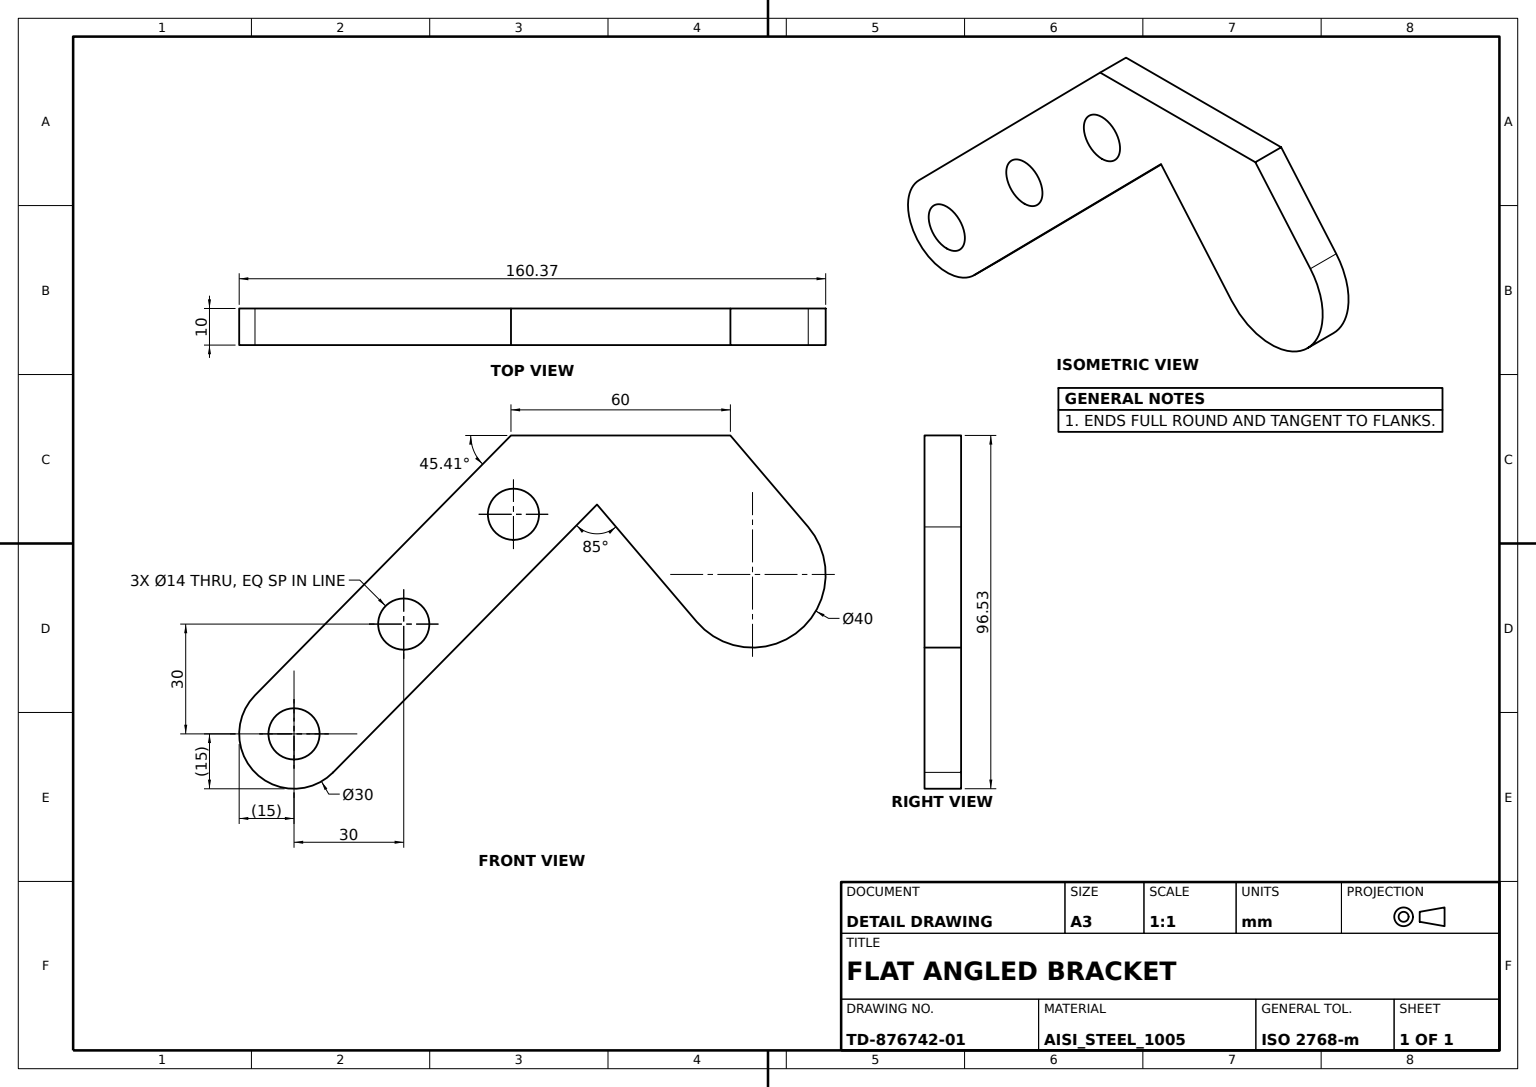
ISO-10303-21;
HEADER;
FILE_DESCRIPTION((''),'2;1');
FILE_NAME('','',(''),(''),'','','');
FILE_SCHEMA(('AUTOMOTIVE_DESIGN'));
ENDSEC;
DATA;
#1=APPLICATION_CONTEXT('');
#2=PRODUCT_CONTEXT('',#1,'mechanical');
#3=PRODUCT('','','',(#2));
#4=PRODUCT_DEFINITION_FORMATION('','',#3);
#5=PRODUCT_DEFINITION_CONTEXT('',#1,'design');
#6=PRODUCT_DEFINITION('','',#4,#5);
#7=PRODUCT_DEFINITION_SHAPE('','',#6);
#8=(LENGTH_UNIT()NAMED_UNIT(*)SI_UNIT(.MILLI.,.METRE.));
#9=(NAMED_UNIT(*)PLANE_ANGLE_UNIT()SI_UNIT($,.RADIAN.));
#10=(NAMED_UNIT(*)SI_UNIT($,.STERADIAN.)SOLID_ANGLE_UNIT());
#11=UNCERTAINTY_MEASURE_WITH_UNIT(LENGTH_MEASURE(0.005),#8,'distance_accuracy_value','');
#12=(GEOMETRIC_REPRESENTATION_CONTEXT(3)GLOBAL_UNCERTAINTY_ASSIGNED_CONTEXT((#11))GLOBAL_UNIT_ASSIGNED_CONTEXT((#8,#9,#10))REPRESENTATION_CONTEXT('',''));
#13=CARTESIAN_POINT('',(-37.964085,-6.052113,10.));
#14=VERTEX_POINT('',#13);
#15=CARTESIAN_POINT('',(-37.964085,-66.052113,10.));
#16=VERTEX_POINT('',#15);
#17=DIRECTION('',(0.,-1.,0.));
#18=VECTOR('',#17,1000.);
#19=LINE('',#13,#18);
#20=EDGE_CURVE('',#14,#16,#19,.T.);
#21=ORIENTED_EDGE('',*,*,#20,.F.);
#22=CARTESIAN_POINT('',(-37.964085,-6.052113,0.));
#23=VERTEX_POINT('',#22);
#24=DIRECTION('',(0.,0.,-1.));
#25=VECTOR('',#24,1000.);
#26=LINE('',#13,#25);
#27=EDGE_CURVE('',#14,#23,#26,.T.);
#28=ORIENTED_EDGE('',*,*,#27,.T.);
#29=CARTESIAN_POINT('',(-37.964085,-66.052113,0.));
#30=VERTEX_POINT('',#29);
#31=LINE('',#22,#18);
#32=EDGE_CURVE('',#23,#30,#31,.T.);
#33=ORIENTED_EDGE('',*,*,#32,.T.);
#34=LINE('',#15,#25);
#35=EDGE_CURVE('',#16,#30,#34,.T.);
#36=ORIENTED_EDGE('',*,*,#35,.F.);
#37=EDGE_LOOP('',(#21,#28,#33,#36));
#38=FACE_BOUND('',#37,.T.);
#39=DIRECTION('',(1.,0.,0.));
#40=AXIS2_PLACEMENT_3D('',#13,#39,#24);
#41=PLANE('',#40);
#42=ADVANCED_FACE('',(#38),#41,.F.);
#43=CARTESIAN_POINT('',(20.567028,-95.370555,0.));
#44=VERTEX_POINT('',#43);
#45=CARTESIAN_POINT('',(13.567028,-95.370555,0.));
#46=DIRECTION('',(0.,0.,1.));
#47=AXIS2_PLACEMENT_3D('',#45,#46,#39);
#48=CIRCLE('',#47,7.);
#49=EDGE_CURVE('',#44,#44,#48,.T.);
#50=ORIENTED_EDGE('',*,*,#49,.T.);
#51=EDGE_LOOP('',(#50));
#52=FACE_BOUND('',#51,.T.);
#53=CARTESIAN_POINT('',(50.567028,-125.370555,0.));
#54=VERTEX_POINT('',#53);
#55=CARTESIAN_POINT('',(43.567028,-125.370555,0.));
#56=AXIS2_PLACEMENT_3D('',#55,#46,#39);
#57=CIRCLE('',#56,7.);
#58=EDGE_CURVE('',#54,#54,#57,.T.);
#59=ORIENTED_EDGE('',*,*,#58,.T.);
#60=EDGE_LOOP('',(#59));
#61=FACE_BOUND('',#60,.T.);
#62=CARTESIAN_POINT('',(-9.432972,-65.370555,0.));
#63=VERTEX_POINT('',#62);
#64=CARTESIAN_POINT('',(-16.432972,-65.370555,0.));
#65=AXIS2_PLACEMENT_3D('',#64,#46,#39);
#66=CIRCLE('',#65,7.);
#67=EDGE_CURVE('',#63,#63,#66,.T.);
#68=ORIENTED_EDGE('',*,*,#67,.T.);
#69=EDGE_LOOP('',(#68));
#70=FACE_BOUND('',#69,.T.);
#71=CARTESIAN_POINT('',(33.035915,-136.052113,0.));
#72=VERTEX_POINT('',#71);
#73=CARTESIAN_POINT('',(54.098141,-114.688998,0.));
#74=VERTEX_POINT('',#73);
#75=CIRCLE('',#56,15.);
#76=EDGE_CURVE('',#72,#74,#75,.T.);
#77=ORIENTED_EDGE('',*,*,#76,.F.);
#78=DIRECTION('',(0.712103814,-0.702074183,0.));
#79=VECTOR('',#78,1000.);
#80=LINE('',#29,#79);
#81=EDGE_CURVE('',#30,#72,#80,.T.);
#82=ORIENTED_EDGE('',*,*,#81,.F.);
#83=ORIENTED_EDGE('',*,*,#32,.F.);
#84=CARTESIAN_POINT('',(-12.964085,15.22933,0.));
#85=VERTEX_POINT('',#84);
#86=DIRECTION('',(-0.761466515,-0.648204247,0.));
#87=VECTOR('',#86,1000.);
#88=LINE('',#84,#87);
#89=EDGE_CURVE('',#85,#23,#88,.T.);
#90=ORIENTED_EDGE('',*,*,#89,.F.);
#91=CARTESIAN_POINT('',(12.964085,-15.22933,0.));
#92=VERTEX_POINT('',#91);
#93=CARTESIAN_POINT('',(0.,0.,0.));
#94=AXIS2_PLACEMENT_3D('',#93,#46,#39);
#95=CIRCLE('',#94,20.);
#96=EDGE_CURVE('',#92,#85,#95,.T.);
#97=ORIENTED_EDGE('',*,*,#96,.F.);
#98=CARTESIAN_POINT('',(-19.098741,-42.523058,0.));
#99=VERTEX_POINT('',#98);
#100=DIRECTION('',(0.761466515,0.648204247,0.));
#101=VECTOR('',#100,1000.);
#102=LINE('',#98,#101);
#103=EDGE_CURVE('',#99,#92,#102,.T.);
#104=ORIENTED_EDGE('',*,*,#103,.F.);
#105=DIRECTION('',(-0.712103814,0.702074183,0.));
#106=VECTOR('',#105,1000.);
#107=LINE('',#73,#106);
#108=EDGE_CURVE('',#74,#99,#107,.T.);
#109=ORIENTED_EDGE('',*,*,#108,.F.);
#110=EDGE_LOOP('',(#77,#82,#83,#90,#97,#104,#109));
#111=FACE_BOUND('',#110,.T.);
#112=PLANE('',#94);
#113=ADVANCED_FACE('',(#52,#61,#70,#111),#112,.F.);
#114=CARTESIAN_POINT('',(54.098141,-114.688998,10.));
#115=VERTEX_POINT('',#114);
#116=CARTESIAN_POINT('',(-19.098741,-42.523058,10.));
#117=VERTEX_POINT('',#116);
#118=LINE('',#114,#106);
#119=EDGE_CURVE('',#115,#117,#118,.T.);
#120=ORIENTED_EDGE('',*,*,#119,.T.);
#121=CARTESIAN_POINT('',(12.964085,-15.22933,10.));
#122=VERTEX_POINT('',#121);
#123=LINE('',#116,#101);
#124=EDGE_CURVE('',#117,#122,#123,.T.);
#125=ORIENTED_EDGE('',*,*,#124,.T.);
#126=CARTESIAN_POINT('',(-12.964085,15.22933,10.));
#127=VERTEX_POINT('',#126);
#128=CARTESIAN_POINT('',(0.,0.,10.));
#129=AXIS2_PLACEMENT_3D('',#128,#46,#39);
#130=CIRCLE('',#129,20.);
#131=EDGE_CURVE('',#122,#127,#130,.T.);
#132=ORIENTED_EDGE('',*,*,#131,.T.);
#133=LINE('',#126,#87);
#134=EDGE_CURVE('',#127,#14,#133,.T.);
#135=ORIENTED_EDGE('',*,*,#134,.T.);
#136=ORIENTED_EDGE('',*,*,#20,.T.);
#137=CARTESIAN_POINT('',(33.035915,-136.052113,10.));
#138=VERTEX_POINT('',#137);
#139=LINE('',#15,#79);
#140=EDGE_CURVE('',#16,#138,#139,.T.);
#141=ORIENTED_EDGE('',*,*,#140,.T.);
#142=CARTESIAN_POINT('',(43.567028,-125.370555,10.));
#143=AXIS2_PLACEMENT_3D('',#142,#46,#39);
#144=CIRCLE('',#143,15.);
#145=EDGE_CURVE('',#138,#115,#144,.T.);
#146=ORIENTED_EDGE('',*,*,#145,.T.);
#147=EDGE_LOOP('',(#120,#125,#132,#135,#136,#141,#146));
#148=FACE_BOUND('',#147,.T.);
#149=CARTESIAN_POINT('',(-9.432972,-65.370555,10.));
#150=VERTEX_POINT('',#149);
#151=CARTESIAN_POINT('',(-16.432972,-65.370555,10.));
#152=AXIS2_PLACEMENT_3D('',#151,#46,#39);
#153=CIRCLE('',#152,7.);
#154=EDGE_CURVE('',#150,#150,#153,.T.);
#155=ORIENTED_EDGE('',*,*,#154,.F.);
#156=EDGE_LOOP('',(#155));
#157=FACE_BOUND('',#156,.T.);
#158=CARTESIAN_POINT('',(50.567028,-125.370555,10.));
#159=VERTEX_POINT('',#158);
#160=CIRCLE('',#143,7.);
#161=EDGE_CURVE('',#159,#159,#160,.T.);
#162=ORIENTED_EDGE('',*,*,#161,.F.);
#163=EDGE_LOOP('',(#162));
#164=FACE_BOUND('',#163,.T.);
#165=CARTESIAN_POINT('',(20.567028,-95.370555,10.));
#166=VERTEX_POINT('',#165);
#167=CARTESIAN_POINT('',(13.567028,-95.370555,10.));
#168=AXIS2_PLACEMENT_3D('',#167,#46,#39);
#169=CIRCLE('',#168,7.);
#170=EDGE_CURVE('',#166,#166,#169,.T.);
#171=ORIENTED_EDGE('',*,*,#170,.F.);
#172=EDGE_LOOP('',(#171));
#173=FACE_BOUND('',#172,.T.);
#174=PLANE('',#129);
#175=ADVANCED_FACE('',(#148,#157,#164,#173),#174,.T.);
#176=ORIENTED_EDGE('',*,*,#161,.T.);
#177=EDGE_LOOP('',(#176));
#178=FACE_BOUND('',#177,.T.);
#179=ORIENTED_EDGE('',*,*,#58,.F.);
#180=EDGE_LOOP('',(#179));
#181=FACE_BOUND('',#180,.T.);
#182=DIRECTION('',(-1.,0.,0.));
#183=AXIS2_PLACEMENT_3D('',#142,#24,#182);
#184=CYLINDRICAL_SURFACE('',#183,7.);
#185=ADVANCED_FACE('',(#178,#181),#184,.F.);
#186=ORIENTED_EDGE('',*,*,#49,.F.);
#187=EDGE_LOOP('',(#186));
#188=FACE_BOUND('',#187,.T.);
#189=ORIENTED_EDGE('',*,*,#170,.T.);
#190=EDGE_LOOP('',(#189));
#191=FACE_BOUND('',#190,.T.);
#192=AXIS2_PLACEMENT_3D('',#167,#24,#182);
#193=CYLINDRICAL_SURFACE('',#192,7.);
#194=ADVANCED_FACE('',(#188,#191),#193,.F.);
#195=LINE('',#121,#25);
#196=EDGE_CURVE('',#122,#92,#195,.T.);
#197=ORIENTED_EDGE('',*,*,#196,.T.);
#198=ORIENTED_EDGE('',*,*,#96,.T.);
#199=LINE('',#126,#25);
#200=EDGE_CURVE('',#127,#85,#199,.T.);
#201=ORIENTED_EDGE('',*,*,#200,.F.);
#202=ORIENTED_EDGE('',*,*,#131,.F.);
#203=EDGE_LOOP('',(#197,#198,#201,#202));
#204=FACE_BOUND('',#203,.T.);
#205=AXIS2_PLACEMENT_3D('',#128,#24,#182);
#206=CYLINDRICAL_SURFACE('',#205,20.);
#207=ADVANCED_FACE('',(#204),#206,.T.);
#208=LINE('',#114,#25);
#209=EDGE_CURVE('',#115,#74,#208,.T.);
#210=ORIENTED_EDGE('',*,*,#209,.T.);
#211=ORIENTED_EDGE('',*,*,#108,.T.);
#212=LINE('',#116,#25);
#213=EDGE_CURVE('',#117,#99,#212,.T.);
#214=ORIENTED_EDGE('',*,*,#213,.F.);
#215=ORIENTED_EDGE('',*,*,#119,.F.);
#216=EDGE_LOOP('',(#210,#211,#214,#215));
#217=FACE_BOUND('',#216,.T.);
#218=DIRECTION('',(-0.702074183,-0.712103814,0.));
#219=AXIS2_PLACEMENT_3D('',#114,#218,#78);
#220=PLANE('',#219);
#221=ADVANCED_FACE('',(#217),#220,.F.);
#222=ORIENTED_EDGE('',*,*,#124,.F.);
#223=ORIENTED_EDGE('',*,*,#213,.T.);
#224=ORIENTED_EDGE('',*,*,#103,.T.);
#225=ORIENTED_EDGE('',*,*,#196,.F.);
#226=EDGE_LOOP('',(#222,#223,#224,#225));
#227=FACE_BOUND('',#226,.T.);
#228=DIRECTION('',(-0.648204247,0.761466515,0.));
#229=AXIS2_PLACEMENT_3D('',#116,#228,#86);
#230=PLANE('',#229);
#231=ADVANCED_FACE('',(#227),#230,.F.);
#232=ORIENTED_EDGE('',*,*,#89,.T.);
#233=ORIENTED_EDGE('',*,*,#27,.F.);
#234=ORIENTED_EDGE('',*,*,#134,.F.);
#235=ORIENTED_EDGE('',*,*,#200,.T.);
#236=EDGE_LOOP('',(#232,#233,#234,#235));
#237=FACE_BOUND('',#236,.T.);
#238=DIRECTION('',(0.648204247,-0.761466515,0.));
#239=AXIS2_PLACEMENT_3D('',#126,#238,#100);
#240=PLANE('',#239);
#241=ADVANCED_FACE('',(#237),#240,.F.);
#242=ORIENTED_EDGE('',*,*,#67,.F.);
#243=EDGE_LOOP('',(#242));
#244=FACE_BOUND('',#243,.T.);
#245=ORIENTED_EDGE('',*,*,#154,.T.);
#246=EDGE_LOOP('',(#245));
#247=FACE_BOUND('',#246,.T.);
#248=AXIS2_PLACEMENT_3D('',#151,#24,#182);
#249=CYLINDRICAL_SURFACE('',#248,7.);
#250=ADVANCED_FACE('',(#244,#247),#249,.F.);
#251=LINE('',#137,#25);
#252=EDGE_CURVE('',#138,#72,#251,.T.);
#253=ORIENTED_EDGE('',*,*,#252,.T.);
#254=ORIENTED_EDGE('',*,*,#76,.T.);
#255=ORIENTED_EDGE('',*,*,#209,.F.);
#256=ORIENTED_EDGE('',*,*,#145,.F.);
#257=EDGE_LOOP('',(#253,#254,#255,#256));
#258=FACE_BOUND('',#257,.T.);
#259=CYLINDRICAL_SURFACE('',#183,15.);
#260=ADVANCED_FACE('',(#258),#259,.T.);
#261=ORIENTED_EDGE('',*,*,#81,.T.);
#262=ORIENTED_EDGE('',*,*,#252,.F.);
#263=ORIENTED_EDGE('',*,*,#140,.F.);
#264=ORIENTED_EDGE('',*,*,#35,.T.);
#265=EDGE_LOOP('',(#261,#262,#263,#264));
#266=FACE_BOUND('',#265,.T.);
#267=DIRECTION('',(0.702074183,0.712103814,0.));
#268=AXIS2_PLACEMENT_3D('',#15,#267,#105);
#269=PLANE('',#268);
#270=ADVANCED_FACE('',(#266),#269,.F.);
#271=CLOSED_SHELL('',(#42,#113,#175,#185,#194,#207,#221,#231,#241,#250,#260,#270));
#272=MANIFOLD_SOLID_BREP('',#271);
#273=ADVANCED_BREP_SHAPE_REPRESENTATION('',(#272),#12);
#274=SHAPE_DEFINITION_REPRESENTATION(#7,#273);
ENDSEC;
END-ISO-10303-21;
